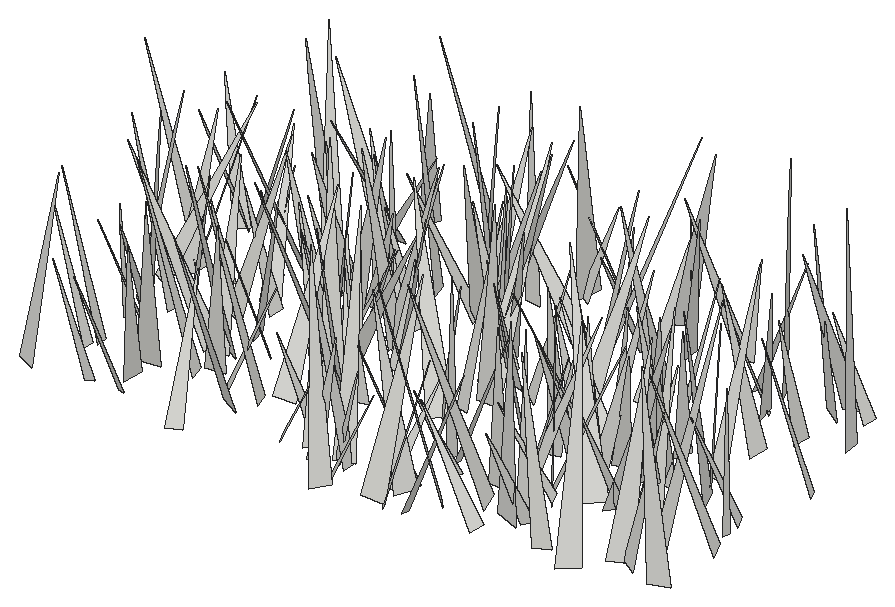
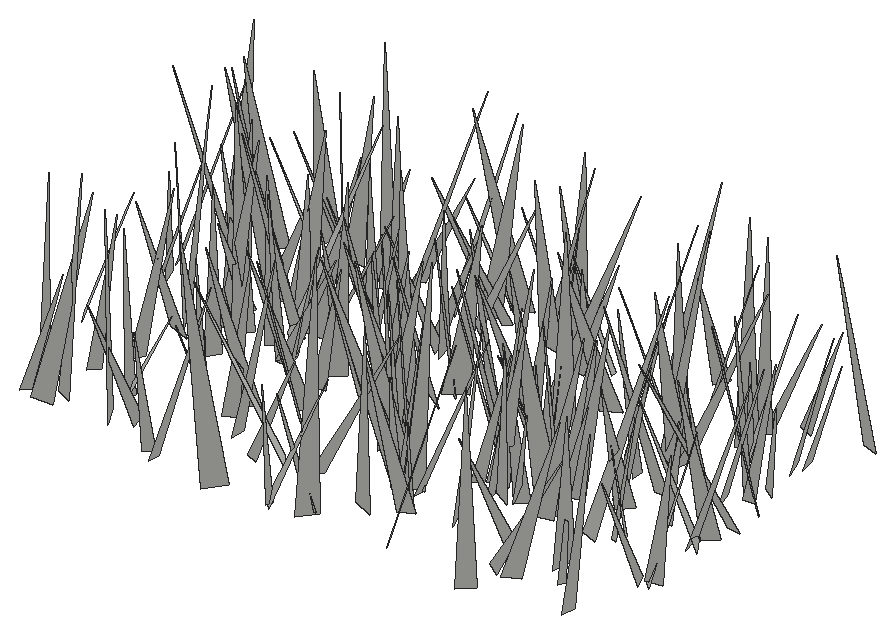
# SketchUp Ruby script. Lengths in inches.
U = 1.inch
M = Sketchup.active_model
def pt(a) = Geom::Point3d.new(a.map { |v| v * U })
def face(e, loops, mat)
  f = e.add_face(loops[0].map { |a| pt(a) })
  loops[1..].each { |l| e.add_face(l.map { |a| pt(a) }).erase! }
  f.material = f.back_material = mat if mat
  f
end
# faces: each face lists its corners as indices into pts; further lists are holes
def faces(e, pts, list, mat = nil) = list.each { |f| face(e, (f[0].is_a?(Array) ? f : [f]).map { |l| l.map { |i| pts[i] } }, mat) }
# xy, xz, yz: faces in a plane at the given z, y or x. An outline is a flat list of corners, or four numbers for a rectangle; further outlines are holes
def ring(l) = l.size == 4 ? [[l[0], l[1]], [l[2], l[1]], [l[2], l[3]], [l[0], l[3]]] : l.each_slice(2).to_a
def flat(e, list, mat, &to3) = list.each { |f| face(e, (f[0].is_a?(Array) ? f : [f]).map { |l| ring(l).map { |u, v| to3.(u, v) } }, mat) }
def xy(e, z, list, mat = nil) = flat(e, list, mat) { |x, y| [x, y, z] }
def xz(e, y, list, mat = nil) = flat(e, list, mat) { |x, z| [x, y, z] }
def yz(e, x, list, mat = nil) = flat(e, list, mat) { |y, z| [x, y, z] }
def lines(e, pts, list) = list.each { |a, b| e.add_line(pt(pts[a]), pt(pts[b])) }
# prism: a flat outline (further loops are holes) pulled along v
def prism(e, loops, v, mat = nil)
  f = face(e, loops, mat); d = Geom::Vector3d.new(v.map { |x| x * U })
  f.pushpull(f.normal.samedirection?(d) ? d.length : -d.length)
end
def box(e, o, s, mat = nil) = prism(e, [[o, [o[0] + s[0], o[1], o[2]], [o[0] + s[0], o[1] + s[1], o[2]], [o[0], o[1] + s[1], o[2]]]], [0, 0, s[2]], mat)
def at(x, y, z, deg = 0) = Geom::Transformation.translation(pt([x, y, z])) * Geom::Transformation.rotation(ORIGIN, Z_AXIS, deg.degrees)
def axes(o, x, y, z) = Geom::Transformation.new([*x, 0, *y, 0, *z, 0, *pt(o).to_a, 1])
def part(name) = M.definitions.add(name)
# library, detail: a bought-in or finely detailed component or shape, given as its bounding box
def library(name, o, s) = part(name).tap { |d| box(d.entities, o, s) }
def detail(e, o, s) = box(e.add_group.entities, o, s)
def put(e, d, t, mat = nil) = e.add_instance(d, t).tap { |i| i.material = mat if mat }
def group(e, t, mat = nil) = e.add_group.tap { |g| g.transformation = t; g.material = mat if mat }.entities
root = M.entities
c1 = part("fur_instance\#9")
p = [[0.8125,0,1.79],[0.67,-0.02,1.48],[0,-0.11,0],[0,0.11,0]]
faces(c1.entities,p,[[0,1,2,3]])
put(root,c1,axes([478.4,355.11,-21.66],[3.77978,1.93812,0.15141],[1.88384,-3.56988,-1.33157],[0.48001,-1.25124,4.0336]))
put(root,c1,axes([461.59,355.39,-21.66],[-2.18116,-3.44946,0.52539],[-3.41914,1.9894,-1.13316],[-0.6959,1.0372,3.92074]))
put(root,c1,axes([454.67,354.57,-21.66],[2.76981,6.05425,2.08045],[6.39697,-2.70498,-0.64491],[-0.24704,-2.16406,6.62646]))
put(root,c1,axes([459.19,355.25,-21.66],[-0.15517,3.72025,1.9318],[3.94772,-0.52047,1.31942],[-1.40985,-1.86683,3.48188]))
put(root,c1,axes([489.59,355.57,-21.66],[-4.14397,2.00475,0.46664],[2.04964,3.92263,1.34951],[-0.1891,-1.41534,4.40117]))
put(root,c1,axes([478.7,353.66,-21.66],[-7.32985,2.37013,1.25415],[2.21242,7.40801,-1.06942],[1.51512,0.64882,7.62892]))
put(root,c1,axes([476.6,355.71,-21.66],[0.64184,-5.02818,1.67754],[-5.1921,-0.25617,1.21871],[1.0672,1.77778,4.9203]))
put(root,c1,axes([461.03,357.24,-21.66],[5.82388,-2.11588,0.96568],[-1.89422,-5.82584,-1.34106],[-1.34958,-0.95373,6.04946]))
put(root,c1,axes([467.08,353.73,-21.66],[-3.56448,3.67904,0.44666],[3.56023,3.5714,-1.00507],[1.02934,0.38746,5.02301]))
put(root,c1,axes([467.98,358.13,-21.66],[-2.86218,-6.85746,0.77217],[-6.83354,2.93291,0.71683],[0.96112,0.43167,7.39614]))
put(root,c1,axes([482.29,354.38,-21.66],[-1.03239,7.59334,1.92082],[7.72051,1.31303,-1.04105],[1.31985,-1.74108,7.59215]))
put(root,c1,axes([483.31,356.38,-21.66],[-5.98098,3.27291,2.42019],[3.72115,6.13978,0.89298],[1.64993,-1.98304,6.75918]))
put(root,c1,axes([484.82,354.41,-21.66],[4.77629,1.47467,0.59608],[1.29577,-4.70156,1.24867],[-0.92247,1.03128,4.84029]))
put(root,c1,axes([483.25,354.15,-21.66],[3.76197,3.17485,0.58422],[2.97684,-3.75885,1.25811],[-1.24876,0.60394,4.75913]))
put(root,c1,axes([485.8,356.79,-21.66],[-5.67662,-5.13617,1.32256],[-5.29359,5.60645,-0.94818],[0.32758,1.59402,7.59639]))
put(root,c1,axes([490.38,357.52,-21.66],[-1.23371,-7.71978,2.49826],[-7.92295,1.69122,1.31342],[1.75022,2.21429,7.70662]))
put(root,c1,axes([494.3125,356.08,-21.66],[-1.23354,6.12021,2.2306],[6.48252,0.93032,1.03231],[-0.63996,-2.37312,6.15735]))
put(root,c1,axes([491.61,358.08,-21.66],[1.92833,-3.54748,0.58332],[-3.33012,-2.01195,-1.22706],[-1.35468,-0.10385,3.84674]))
put(root,c1,axes([477.5,356.91,-21.66],[2.1321,2.91958,1.28602],[3.18698,-1.87905,-1.01782],[0.14466,-1.63367,3.46899]))
put(root,c1,axes([472.9375,357.05,-21.66],[3.88446,1.51086,0.00017],[1.46105,-3.75628,-1.06181],[0.38475,-0.98965,4.03042]))
put(root,c1,axes([502.85,356.97,-21.66],[1.15068,-6.84996,3.27998],[-7.48842,-1.57649,-0.66528],[-1.26644,3.09791,6.914]))
put(root,c1,axes([488.1,358.59,-21.66],[-7.76303,-2.55675,1.09489],[-2.43873,7.81802,0.96517],[1.33728,-0.58482,8.11604]))
put(root,c1,axes([483.13,357.85,-21.66],[-3.10953,-4.00727,0.37973],[-3.98696,3.00024,-0.98706],[-0.55366,0.90108,4.97525]))
put(root,c1,axes([460.71,359.18,-21.66],[2.24537,-6.9608,0.71668],[-6.96969,-2.1575,0.8813],[0.62434,0.94895,7.26069]))
put(root,c1,axes([497.1,355.2,-21.66],[5.53383,-2.65462,5.00816],[-4.23304,-6.59023,1.18414],[-3.76962,3.5034,6.0223]))
put(root,c1,axes([478.58,356.73,-21.66],[-7.60093,-1.69118,1.08047],[-1.85126,7.54274,-1.21718],[0.77483,1.43129,7.69108]))
put(root,c1,axes([481.97,356.27,-21.66],[0.26684,4.21608,0.5662],[4.07293,-0.08948,-1.25314],[1.22767,-0.6195,4.03438]))
put(root,c1,axes([474.83,358.29,-21.66],[0.84597,-3.78981,1.14812],[-3.67965,-1.18614,-1.20406],[-1.46323,0.79177,3.69169]))
put(root,c1,axes([499.85,357.69,-21.66],[3.01267,4.99828,1.819],[5.31773,-2.78497,-1.15474],[0.11548,-2.15148,5.72063]))
put(root,c1,axes([475.11,357.125,-21.66],[-3.68366,1.92684,0.76086],[1.83141,3.75443,-0.64122],[0.96827,0.22919,4.10742]))
put(root,c1,axes([484.4,360.06,-21.66],[1.61464,-3.26071,0.69447],[-2.99454,-1.75765,-1.29032],[-1.46534,-0.00102,3.40211]))
put(root,c1,axes([456.35,358.68,-21.66],[-4.63616,-0.58897,0.33378],[-0.62989,4.59941,-0.63319],[0.24806,0.67142,4.63033]))
put(root,c1,axes([499.08,357.76,-21.66],[-4.71435,5.59524,2.23508],[5.56124,5.13291,-1.11952],[2.31839,-0.93486,7.23039]))
put(root,c1,axes([487.35,360.49,-21.66],[0.93072,-6.54849,1.55591],[-6.7031,-0.75944,0.81335],[0.60996,1.64631,6.5641]))
put(root,c1,axes([477.91,357.04,-21.66],[-0.32528,8.12923,0.88129],[8.06717,0.17507,1.36272],[-1.33486,-0.92294,8.0208]))
put(root,c1,axes([459.21,361.34,-21.66],[-3.58338,-3.97137,0.418],[-3.89573,3.60001,0.80641],[0.87736,-0.23507,5.28792]))
put(root,c1,axes([464.53,361.03,-21.66],[2.07468,-5.92746,1.15005],[-6.03286,-1.98482,0.6533],[0.24901,1.299,6.24598]))
put(root,c1,axes([466.5,359.74,-21.66],[3.8277,2.64651,0.3376],[2.6435,-3.68235,-1.10521],[0.36045,-1.09797,4.52038]))
put(root,c1,axes([456.77,359.47,-21.66],[-5.59376,-1.56322,0.76508],[-1.67452,5.53596,-0.93185],[0.47433,1.10847,5.73284]))
put(root,c1,axes([469.09,359.85,-21.66],[-7.24522,-3.15461,1.03201],[-3.28219,7.17812,-1.10079],[0.49381,1.42581,7.82516]))
put(root,c1,axes([463.77,360.12,-21.66],[-6.93543,-2.32629,0.88421],[-2.41004,6.93097,-0.66862],[0.62063,0.91853,7.28456]))
put(root,c1,axes([490.93,361.54,-21.66],[-3.84083,-1.16764,0.10273],[-1.10793,3.73134,0.98769],[0.38264,-0.91633,3.89099]))
put(root,c1,axes([490,359.65,-21.66],[1.00537,5.49165,1.69021],[5.63183,-1.28199,0.81538],[-1.13911,-1.49133,5.52306]))
put(root,c1,axes([490.86,361.4,-21.66],[5.50119,4.10651,2.99111],[4.73487,-5.74232,-0.82461],[-1.84151,-2.49711,6.81516]))
put(root,c1,axes([502.91,362.64,-21.66],[-6.09562,-2.74651,0.83103],[-2.67616,6.14538,0.68045],[1.03541,-0.28555,6.65108]))
put(root,c1,axes([473.25,362.97,-21.66],[-4.28269,-7.03673,0.88853],[-7.06243,4.13524,-1.29164],[-0.65353,1.42504,8.13564]))
put(root,c1,axes([495.52,362.71,-21.66],[-0.21744,-4.53269,0.61909],[-4.46943,0.07824,-0.99696],[-0.9761,0.65149,4.42703]))
put(root,c1,axes([463.72,363.48,-21.66],[-3.21608,-6.87634,1.40534],[-6.91778,3.36666,0.64196],[1.18463,0.99184,7.56406]))
put(root,c1,axes([459.44,360.45,-21.66],[-4.54245,-0.30979,1.16713],[-0.64985,4.4561,-1.34644],[1.01777,1.46262,4.34936]))
put(root,c1,axes([489.15,360.64,-21.66],[3.76049,3.04894,0.61025],[2.98388,-3.80785,0.6375],[-0.87456,0.11813,4.79905]))
put(root,c1,axes([489.02,361.08,-21.66],[3.55811,5.92159,0.8478],[5.93377,-3.36884,-1.37307],[0.75783,-1.4247,6.77052]))
put(root,c1,axes([482.8,361.5,-21.66],[-5.66532,-0.50223,1.85308],[-0.88322,5.80808,-1.12609],[1.70472,1.34012,5.57494]))
put(root,c1,axes([483.44,361.32,-21.66],[4.63443,1.21877,0.59299],[1.09033,-4.6073,0.94811],[-0.80513,0.77609,4.69728]))
put(root,c1,axes([494.73,362.78,-21.66],[7.07738,-3.29601,0.99897],[-3.4049,-7.03943,0.89669],[-0.51794,1.23844,7.75557]))
put(root,c1,axes([462.375,363.35,-21.66],[-7.38136,0.22251,0.33251],[0.26326,7.32737,0.9407],[0.30128,-0.95116,7.32455]))
put(root,c1,axes([456.39,364.4,-21.66],[-0.44013,-4.40012,0.04518],[-4.35564,0.44209,0.62427],[0.62566,-0.01764,4.37779]))
put(root,c1,axes([490.32,362.11,-21.66],[5.45999,3.37552,0.2587],[3.37248,-5.38033,-0.97518],[0.29572,-0.96459,6.34466]))
put(root,c1,axes([496.49,364.54,-21.66],[1.50872,-5.62418,0.24688],[-5.60162,-1.47433,0.64555],[0.56049,0.40439,5.78713]))
put(root,c1,axes([472.18,363.84,-21.66],[4.90048,2.76624,3.25214],[3.64641,-5.28694,-0.99757],[-2.22086,-2.5767,5.5382]))
put(root,c1,axes([490.55,364.79,-21.66],[1.73584,-5.70606,0.92261],[-5.63591,-1.88469,-1.0526],[-1.28332,0.55882,5.87063]))
put(root,c1,axes([465.66,364.84,-21.66],[-3.10311,-4.08719,0.56583],[-3.96021,3.14894,1.02739],[1.15846,-0.18348,5.02781]))
put(root,c1,axes([499.88,360.8,-21.66],[3.85814,7.37241,1.12129],[7.37277,-3.96052,0.67189],[-1.11889,-0.67587,8.29374]))
put(root,c1,axes([470.13,360.82,-21.66],[-2.04424,6.85145,0.72305],[6.79433,2.1298,-0.97223],[1.1412,-0.40704,7.08351]))
put(root,c1,axes([456.1,362.78,-21.66],[1.10778,3.32388,1.25845],[3.28018,-1.46364,0.97838],[-1.36832,-0.8177,3.36424]))
put(root,c1,axes([491.39,366.02,-21.66],[-5.30348,-5.59312,0.1785],[-5.55783,5.29332,0.73008],[0.65218,-0.37354,7.67313]))
put(root,c1,axes([474.1875,363.45,-21.66],[-0.90978,-4.59674,2.27002],[-5.08569,0.51819,-0.98893],[-0.64715,2.39002,4.58036]))
put(root,c1,axes([463.36,362.65,-21.66],[-4.06355,5.05875,1.67662],[5.05755,4.32523,-0.79246],[1.68023,-0.78477,6.44014]))
put(root,c1,axes([493.18,362.65,-21.66],[-5.00695,6.61488,0.9269],[6.67749,4.92855,0.89773],[-0.16413,-1.27989,8.24744]))
put(root,c1,axes([492.35,363.61,-21.66],[-0.54447,5.56352,1.73211],[5.79599,0.33809,0.73596],[-0.59958,-1.78391,5.54144]))
put(root,c1,axes([457.49,363.17,-21.66],[-6.13991,-1.94187,2.86824],[-2.65031,6.39227,-1.34568],[2.23013,2.25037,6.2975]))
put(root,c1,axes([501.75,366.36,-21.66],[-4.09527,-2.1175,0.66115],[-1.87882,4.04889,1.32991],[1.17939,-0.90267,4.41434]))
put(root,c1,axes([478.91,365.37,-21.66],[3.62429,3.41254,1.71474],[3.78655,-3.51895,-1.00013],[-0.49783,-1.92166,4.87654]))
put(root,c1,axes([495.22,367.21,-21.66],[5.27759,-3.33069,0.22963],[-3.2336,-5.20637,-1.19863],[-0.83073,-0.89406,6.12452]))
put(root,c1,axes([485.89,365,-21.66],[-3.65286,-4.07637,1.60167],[-4.37583,3.48496,-1.11027],[0.18514,1.94004,5.3598]))
put(root,c1,axes([497.68,362.94,-21.66],[0.68594,6.83231,0.78357],[6.74689,-0.82108,1.2531],[-1.33188,-0.64057,6.75135]))
put(root,c1,axes([471.09,364.36,-21.66],[-7.16118,3.19135,1.99245],[3.1192,7.43157,-0.69239],[2.1036,-0.15533,7.80947]))
put(root,c1,axes([487.46,365.8,-21.66],[2.40925,-3.29701,1.00546],[-3.44676,-2.29271,0.74099],[0.03277,1.24857,4.01568]))
put(root,c1,axes([502.13,364.55,-21.66],[-4.48133,-0.60292,1.35721],[-0.97091,4.45413,-1.22715],[1.12377,1.44397,4.35201]))
put(root,c1,axes([463.83,366.14,-21.66],[5.32416,0.8497,1.29821],[1.01973,-5.41351,-0.63884],[-1.1694,-0.85204,5.35356]))
put(root,c1,axes([494.05,367.3125,-21.66],[6.83248,-2.68093,1.04491],[-2.55055,-6.88917,-0.99801],[-1.33189,-0.56029,7.27146]))
put(root,c1,axes([498.56,367.18,-21.66],[-6.30807,-3.21691,2.7037],[-2.95993,6.86307,1.25992],[2.98285,0.00727,6.96799]))
put(root,c1,axes([491.66,367.25,-21.66],[2.32363,-4.81619,0.47979],[-4.81966,-2.25368,0.71896],[0.44354,0.74187,5.29887]))
put(root,c1,axes([457.63,365.42,-21.66],[-6.22819,-1.34042,0.61243],[-1.44458,6.07908,-1.38568],[0.29149,1.48668,6.21828]))
put(root,c1,axes([478.98,365.13,-21.66],[-5.24663,5.623,0.95369],[5.70188,5.20042,0.70642],[0.12741,-1.17997,7.65808]))
put(root,c1,axes([495.56,367.01,-21.66],[0.0044,-6.27087,2.13822],[-6.5778,-0.25997,-0.7489],[-0.79272,2.12236,6.226]))
put(root,c1,axes([455.375,364.86,-21.66],[4.64173,5.41011,1.53464],[5.42173,-4.8336,0.64123],[-1.49305,-0.73288,7.09956]))
put(root,c1,axes([459.18,365.27,-21.66],[-4.14484,-0.82966,2.07391],[-1.4546,4.32013,-1.17886],[1.69516,1.67847,4.05935]))
put(root,c1,axes([491.34,365.32,-21.66],[2.79902,6.82497,1.56007],[7.00009,-2.70115,-0.74237],[0.11309,-1.72399,7.33919]))
put(root,c1,axes([486.125,367.95,-21.66],[4.8862,-3.80667,1.31151],[-3.74132,-5.05482,-0.73291],[-1.48774,0.20937,6.1505]))
put(root,c1,axes([474.12,367.01,-21.66],[6.26752,1.77798,1.53658],[2.00319,-6.33057,-0.84565],[-1.22862,-1.25168,6.45971]))
put(root,c1,axes([495.37,365.12,-21.66],[-3.3116,2.69695,0.72945],[2.42136,3.33487,-1.33716],[1.39378,0.61437,4.05614]))
put(root,c1,axes([468.21,366.48,-21.66],[-1.43576,4.62376,1.24523],[4.74317,1.1948,1.0324],[-0.65727,-1.47798,4.73019]))
put(root,c1,axes([480.35,368.27,-21.66],[1.05516,-7.50337,2.43147],[-7.87164,-0.84629,0.8044],[0.49989,2.51181,7.53438]))
put(root,c1,axes([470.29,367.33,-21.66],[5.56558,-2.4926,0.3103],[-2.49513,-5.39934,1.38077],[0.28926,1.38533,5.93988]))
put(root,c1,axes([467.14,369.09,-21.66],[-3.93498,0.71077,2.15609],[1.47172,4.08376,1.33974],[1.72857,-1.85895,3.76754]))
put(root,c1,axes([461.14,367.06,-21.66],[2.20928,6.37096,1.50715],[6.50914,-1.9672,-1.22586],[0.70121,-1.81177,6.63078]))
put(root,c1,axes([473.26,367.99,-21.66],[-1.45732,3.49071,1.72371],[3.67662,1.83923,-0.61623],[1.28012,-1.30851,3.73217]))
put(root,c1,axes([462.875,369.07,-21.66],[-4.43499,0.78648,1.49873],[1.10021,4.53377,0.87655],[1.28619,-1.16631,4.41807]))
put(root,c1,axes([470.23,367.0625,-21.66],[-1.23415,4.06964,0.18802],[4.01431,1.18128,0.78126],[-0.69473,-0.40381,4.18028]))
put(root,c1,axes([489.87,368.8,-21.66],[-1.04898,-5.12431,2.12616],[-5.35306,1.50327,0.98203],[1.45734,1.83333,5.13756]))
put(root,c1,axes([497.5,368.81,-21.66],[5.0794,2.90769,2.21904],[3.29641,-5.28463,-0.62087],[-1.58507,-1.67247,5.81975]))
put(root,c1,axes([458.54,369.92,-21.66],[3.22144,-2.0672,0.86258],[-1.86043,-3.31076,-0.98626],[-1.24746,-0.40075,3.69841]))
put(root,c1,axes([489.88,368.5,-21.66],[-3.98181,3.20015,0.16473],[3.12043,3.81261,1.36007],[-0.7287,-1.16015,4.92402]))
put(root,c1,axes([489.4,368.14,-21.66],[-5.02924,-0.94611,0.83871],[-1.10156,4.96734,-1.00192],[0.62059,1.14984,5.01842]))
put(root,c1,axes([470.28,367.86,-21.66],[3.75823,0.40452,0.85087],[0.18545,-3.74836,0.96295],[-0.9237,0.89332,3.65522]))
put(root,c1,axes([470.07,368.05,-21.66],[-3.57041,1.71359,0.7726],[1.61509,3.64514,-0.62093],[0.96166,0.24019,3.91135]))
put(root,c1,axes([479.47,366.68,-21.66],[2.76869,6.15296,0.77217],[6.00563,-2.8712,1.34513],[-1.54517,-0.13446,6.61174]))
put(root,c1,axes([480.22,371.06,-21.66],[-0.97227,-5.54065,0.71566],[-5.53732,1.05209,0.62249],[0.741,0.5921,5.59077]))
put(root,c1,axes([468.65,368.94,-21.66],[3.29309,2.39527,0.08068],[2.3726,-3.23886,-0.68467],[0.3385,-0.60058,4.0141]))
put(root,c1,axes([486.05,369.91,-21.66],[1.60844,-3.68609,1.55705],[-3.78668,-1.94455,-0.69177],[-1.29334,1.10916,3.96179]))
put(root,c1,axes([493.79,370.66,-21.66],[4.8037,-2.51399,0.9877],[-2.43404,-4.90267,-0.64073],[-1.17095,-0.12226,5.38379]))
put(root,c1,axes([465.04,370.87,-21.66],[3.86572,-4.28586,2.24353],[-4.19582,-4.39988,-1.17556],[-2.40771,0.7863,5.6507]))
put(root,c1,axes([471.23,370.55,-21.66],[-6.84332,-0.22544,2.15666],[-0.013,7.14388,0.70553],[2.16837,-0.66867,6.81058]))
put(root,c1,axes([454.86,367.79,-21.66],[2.4491,6.4359,0.09226],[6.32974,-2.3903,-1.28384],[1.16776,-0.54137,6.7654]))
put(root,c1,axes([455.2,369.65,-21.66],[2.82826,-4.43632,2.67471],[-5.15951,-2.68482,1.00262],[-0.46309,2.81866,5.16476]))
put(root,c1,axes([466.21,370.95,-21.66],[-4.16703,-2.76107,2.92288],[-2.78486,5.0182,0.77013],[2.90022,0.85149,4.93909]))
put(root,c1,axes([467.42,370.69,-21.66],[6.54433,-2.87567,1.841],[-3.10892,-6.66403,0.64215],[-1.41189,1.3447,7.11937]))
put(root,c1,axes([470.91,370.25,-21.66],[3.79421,5.57197,1.64798],[5.81056,-3.63804,-1.07735],[0.00109,-1.96889,6.65448]))
put(root,c1,axes([461.38,374,-21.66],[-3.81436,-7.20009,0.2192],[-7.12697,3.80817,1.069],[1.0467,-0.30859,8.07762]))
put(root,c1,axes([482.01,370.36,-21.66],[2.56604,4.25646,1.10853],[4.39439,-2.42581,-0.85772],[0.18887,-1.38883,4.89555]))
put(root,c1,axes([455.83,370.68,-21.66],[-7.51977,-1.08655,0.44758],[-1.14316,7.43533,-1.15625],[0.27218,1.20961,7.50937]))
put(root,c1,axes([478.6,372.33,-21.66],[3.4747,-4.84053,2.29693],[-4.84614,-4.00697,-1.11322],[-2.28507,1.13736,5.85363]))
put(root,c1,axes([503.1,371.84,-21.66],[-4.74174,-2.50609,0.51828],[-2.55748,4.67952,-0.77105],[0.09149,0.92453,5.30754]))
put(root,c1,axes([470.41,371.08,-21.66],[4.17066,5.06918,1.33611],[5.23853,-4.09478,-0.81653],[-0.19883,-1.55319,6.51339]))
put(root,c1,axes([461.78,369.88,-21.66],[-3.2921,4.67046,0.35788],[4.62081,3.30978,-0.68745],[0.76768,0.10645,5.67261]))
put(root,c1,axes([478.07,373.24,-21.66],[6.05752,-0.57817,0.88939],[-0.39,-6.0087,-1.2499],[-0.9865,-1.17476,5.9553]))
put(root,c1,axes([459.88,373.37,-21.66],[-2.01295,-3.23513,0.63988],[-3.06607,2.112,1.03257],[1.21439,-0.03018,3.66768]))
put(root,c1,axes([467.22,373.29,-21.66],[2.01974,-4.62687,0.27657],[-4.52399,-1.90214,1.21619],[1.00891,0.73329,4.89981]))
put(root,c1,axes([459.48,372.65,-21.66],[4.05743,2.55482,1.17911],[2.80714,-3.81746,-1.3882],[-0.19333,-1.81108,4.58942]))
put(root,c1,axes([471.05,372.89,-21.66],[3.41803,-2.18502,2.15563],[-1.95303,-4.03718,-0.99543],[-2.36786,0.1758,3.93273]))
put(root,c1,axes([465.02,373.96,-21.66],[2.93992,-5.13493,1.13143],[-5.01799,-3.12719,-1.15379],[-1.5708,0.37938,5.8034]))
put(root,c1,axes([464.36,373.19,-21.66],[0.87067,-3.63818,0.96208],[-3.64876,-1.05785,-0.69825],[-0.92116,0.75142,3.67517]))
put(root,c1,axes([455.3125,370.8,-21.66],[5.06961,3.19969,0.78256],[3.08145,-5.11429,0.94868],[-1.16407,0.39664,5.91937]))
put(root,c1,axes([497.24,369.67,-21.66],[1.20703,6.81999,0.05967],[6.70849,-1.19813,1.23829],[-1.22962,0.158,6.81439]))
put(root,c1,axes([469.2,373.92,-21.66],[-5.69321,-2.11736,2.09192],[-1.78965,6.04293,1.24584],[2.37833,-0.52131,5.94506]))
put(root,c1,axes([478.99,370.16,-21.66],[-1.14842,8.02715,0.79991],[8.02073,1.22255,-0.75306],[0.86188,-0.68125,8.07384]))
put(root,c1,axes([478,372,-21.66],[7.83085,1.1219,1.78667],[1.00117,-8.02181,0.64907],[-1.85702,0.40616,7.88414]))
put(root,c1,axes([478.03,372.07,-21.66],[2.88835,4.68484,1.93004],[4.79823,-3.24275,0.69058],[-1.62782,-1.24585,5.46016]))
put(root,c1,axes([469.86,372.42,-21.66],[-2.9661,5.6248,1.68099],[5.86235,2.73802,1.18234],[-0.31135,-2.03143,6.24805]))
put(root,c1,axes([497.25,373.77,-21.66],[-5.83631,0.9789,1.84731],[1.28037,6.00401,0.86359],[1.65271,-1.19453,5.85448]))
put(root,c1,axes([476.66,374.19,-21.66],[6.37942,2.61315,2.43113],[3.05762,-6.56979,-0.96169],[-1.84118,-1.85616,6.82648]))
put(root,c1,axes([473.53,376.09,-21.66],[0.50064,-7.21064,0.91051],[-7.21991,-0.3887,0.89157],[0.83387,0.96363,7.17281]))
put(root,c1,axes([467.76,373.13,-21.66],[-4.02809,-0.22088,0.67447],[-0.39433,3.92835,-1.06856],[0.59008,1.11738,3.89005]))
put(root,c1,axes([488.08,376.04,-21.66],[3.42227,-3.49613,0.30492],[-3.40506,-3.41104,-0.89344],[-0.84941,-0.41195,4.81005]))
put(root,c1,axes([484.82,372.57,-21.66],[0.10942,6.44965,1.02032],[6.44115,0.06102,-1.07648],[1.07264,-1.02435,6.36012]))
put(root,c1,axes([468.54,373.65,-21.66],[2.01081,5.29668,2.07869],[5.40677,-2.46554,1.0522],[-1.77275,-1.51176,5.56697]))
put(root,c1,axes([454.66,376.55,-21.66],[-3.71629,-3.62879,0.54604],[-3.4741,3.72939,1.13989],[1.18191,-0.44788,5.0675]))
put(root,c1,axes([472.95,376.35,-21.66],[-5.60277,-1.40853,0.55452],[-1.25772,5.51462,1.29985],[0.84237,-1.13469,5.62898]))
put(root,c1,axes([474.89,375.5,-21.66],[5.41416,-4.66063,0.97473],[-4.76032,-5.26587,1.26282],[0.1044,1.59183,7.03135]))
put(root,c1,axes([487.88,374.16,-21.66],[-0.68675,5.73435,1.62653],[5.78722,1.03346,-1.2],[1.42703,-1.4315,5.64928]))
put(root,c1,axes([498.39,376.66,-21.66],[4.51587,-1.82573,1.61231],[-1.49442,-4.75873,-1.20297],[-1.92343,-0.58918,4.72009]))
put(root,c1,axes([484.13,373.97,-21.66],[4.06792,5.19434,1.22411],[5.14399,-4.22635,0.83955],[-1.42088,-0.42943,6.54403]))
put(root,c1,axes([454.54,376.09,-21.66],[-2.06507,4.56305,1.47225],[4.79287,1.92061,0.77009],[-0.13147,-1.65628,4.94903]))
put(root,c1,axes([474.97,375.58,-21.66],[7.79072,-0.23447,0.87822],[-0.35324,-7.76347,1.06082],[-0.83754,1.09323,7.72172]))
put(root,c1,axes([486.36,377.47,-21.66],[-6.02473,-0.71032,1.74625],[-0.51818,6.24626,0.75302],[1.81257,-0.57532,6.01954]))
put(root,c1,axes([494.53,377.91,-21.66],[5.27182,0.13194,1.25121],[0.40362,-5.28245,-1.14356],[-1.19165,-1.2055,5.14798]))
put(root,c1,axes([474.9,376.16,-21.66],[-4.32916,0.66549,1.27706],[0.40908,4.44763,-0.93094],[1.38073,0.76884,4.27993]))
put(root,c1,axes([474.12,376.91,-21.66],[-5.98871,-2.33617,1.80164],[-2.60473,6.10133,-0.74665],[1.38529,1.37273,6.38474]))
put(root,c1,axes([472.31,377.81,-21.66],[5.33637,4.77614,2.80857],[5.34994,-5.45601,-0.88678],[-1.44141,-2.56842,7.10647]))
put(root,c1,axes([469.09,377.39,-21.66],[-6.68963,-2.36331,2.10659],[-2.62997,6.88987,-0.62215],[1.76244,1.31094,7.06748]))
put(root,c1,axes([479.42,378.38,-21.66],[-6.11827,1.22354,0.04324],[1.20265,5.96505,1.37981],[-0.22923,-1.36132,6.08493]))
put(root,c1,axes([455.33,376.48,-21.66],[3.79033,1.52401,0.8214],[1.29616,-3.80865,1.0854],[-1.14773,0.73179,3.93842]))
put(root,c1,axes([489.63,376.25,-21.66],[2.15657,3.40289,0.33157],[3.29952,-2.17412,0.8525],[-0.89598,0.18416,3.93747]))
put(root,c1,axes([494.66,378.1,-21.66],[-3.19994,-2.12817,0.10035],[-2.08753,3.09569,-0.91527],[-0.42587,0.81635,3.73243]))
put(root,c1,axes([483.8,379.3,-21.66],[-1.02707,-3.52995,0.46815],[-3.49734,0.90838,-0.82343],[-0.66956,0.66999,3.58293]))
put(root,c1,axes([458.94,379.68,-21.66],[3.4639,-0.21189,1.20284],[0.06017,-3.58323,-0.80448],[-1.21988,-0.7784,3.37584]))
put(root,c1,axes([501.33,377.95,-21.66],[-7.33304,-1.55705,2.53328],[-2.07568,7.50758,-1.39398],[2.1292,1.95633,7.36578]))
put(root,c1,axes([497.77,380.41,-21.66],[-3.27673,-6.38483,2.25273],[-6.55108,3.62196,0.73666],[1.71005,1.64109,7.13865]))
put(root,c1,axes([462.99,378.95,-21.66],[4.12414,-1.44643,0.07491],[-1.4095,-3.95608,1.21201],[0.33327,1.1677,4.19901]))
put(root,c1,axes([486.26,380.72,-21.66],[6.1777,-0.38175,1.16241],[-0.13775,-6.16226,-1.29169],[-1.21571,-1.24165,6.0532]))
put(root,c1,axes([498.44,381.74,-21.66],[1.25653,-6.81976,0.6894],[-6.81087,-1.32116,-0.65555],[-0.77223,0.55558,6.90349]))
put(root,c1,axes([460.31,377.83,-21.66],[-6.55915,2.85076,0.80174],[2.70921,6.56329,-1.17278],[1.19574,0.76707,7.05506]))
put(root,c1,axes([472.05,378.7,-21.66],[-0.35457,5.93898,1.63328],[6.05839,0.63143,-0.98081],[1.11129,-1.54746,5.86815]))
put(root,c1,axes([463.4,380.92,-21.66],[-2.21504,-4.22644,0.02495],[-4.06696,2.12371,-1.31133],[-1.15036,0.62998,4.58799]))
put(root,c1,axes([500.15,381.21,-21.66],[-3.89042,0.9571,1.21715],[1.27935,3.84105,1.06884],[0.87221,-1.36496,3.86121]))
put(root,c1,axes([474.51,379.93,-21.66],[1.78909,6.44129,2.50482],[6.73985,-2.19865,0.83993],[-1.52927,-2.15428,6.63216]))
put(root,c1,axes([461.87,381.08,-21.66],[-5.02266,3.34128,1.54054],[3.64584,4.87057,1.32283],[0.49523,-1.96924,5.88569]))
put(root,c1,axes([476.65,382.77,-21.66],[7.55718,-3.05255,1.8054],[-2.7949,-7.74218,-1.39129],[-2.18313,-0.65505,8.03077]))
put(root,c1,axes([481.8,378.45,-21.66],[5.80303,5.01805,0.27093],[4.96083,-5.78629,0.91567],[-0.80277,0.51711,7.61693]))
put(root,c1,axes([492.18,380.02,-21.66],[4.56042,0.58445,0.815],[0.35248,-4.48653,1.24501],[-0.93891,1.15443,4.42595]))
put(root,c1,axes([456.45,382.18,-21.66],[-5.67591,-0.59927,2.29984],[-0.30227,6.08824,0.84044],[2.35734,-0.66225,5.64524]))
put(root,c1,axes([493.87,380.6875,-21.66],[-6.60957,-3.13791,3.29203],[-3.79035,7.01015,-0.92809],[2.51341,2.31982,7.25752]))
put(root,c1,axes([488.53,383.08,-21.66],[-5.81258,-1.56867,1.18702],[-1.32265,5.85738,1.26392],[1.45614,-0.94136,5.88637]))
put(root,c1,axes([470.77,381.93,-21.66],[-7.3033,-3.33888,1.09507],[-3.45877,7.27632,-0.88176],[0.61989,1.26191,7.98178]))
put(root,c1,axes([463.27,383.8,-21.66],[5.23311,-3.59302,0.50013],[-3.53385,-5.24745,-0.7222],[-0.81967,-0.31597,6.30664]))
put(root,c1,axes([483.375,383.49,-21.66],[5.39011,-5.98506,0.75501],[-6.02641,-5.29691,1.03406],[0.27067,1.25142,7.9878]))
put(root,c1,axes([479.37,383.11,-21.66],[3.73813,0.01426,0.67221],[0.17612,-3.68545,-0.90117],[-0.64889,-0.91811,3.62791]))
put(root,c1,axes([476.63,382.3,-21.66],[-0.2038,-3.57727,1.86557],[-3.68837,0.92217,1.36537],[1.63497,1.63446,3.31273]))
put(root,c1,axes([479.48,383.09,-21.66],[-3.75562,-3.58045,0.3486],[-3.58145,3.67402,-0.84892],[-0.33818,0.85312,5.11895]))
put(root,c1,axes([489.34,382.5625,-21.66],[1.31397,-3.56018,1.31098],[-3.78942,-1.16427,0.63629],[0.18405,1.44556,3.7412]))
put(root,c1,axes([484.41,383.1,-21.66],[3.50873,2.55931,1.93983],[3.03472,-3.58228,-0.76287],[-1.05048,-1.80039,4.27543]))
